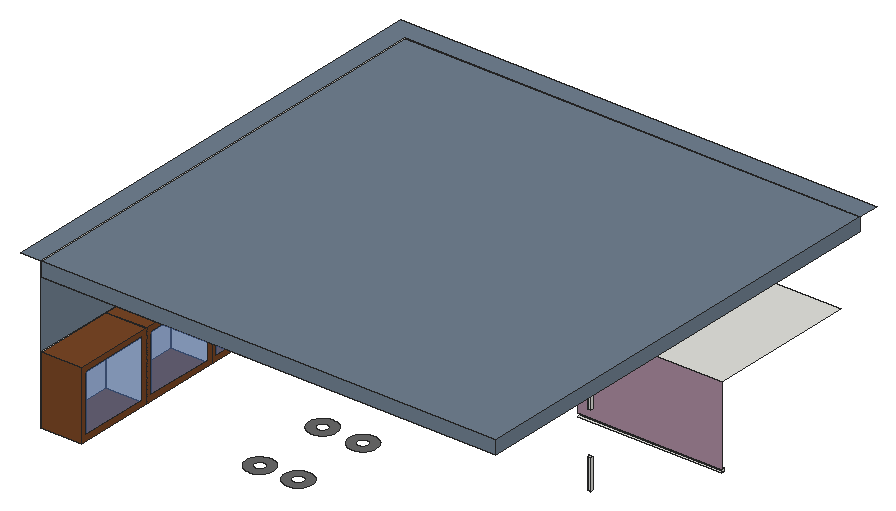
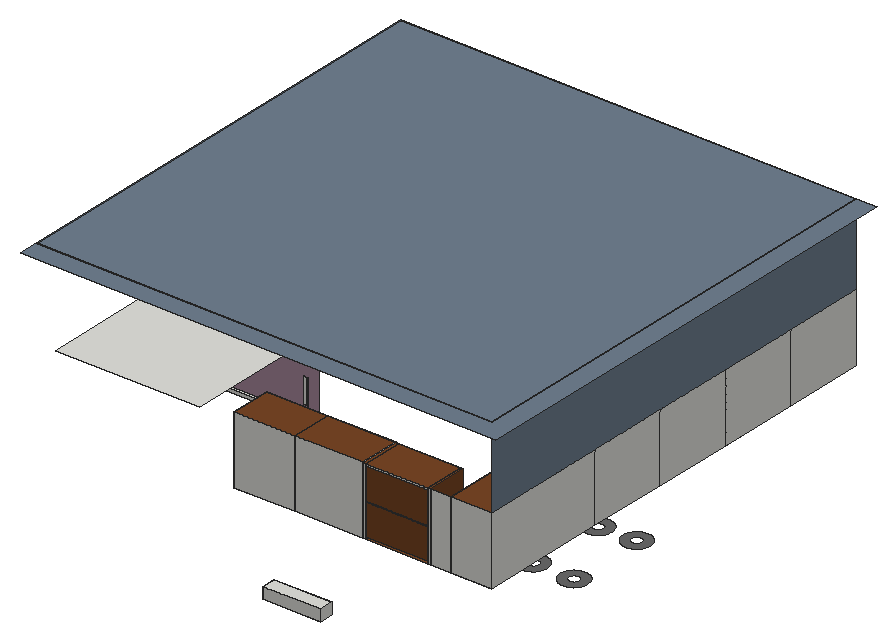
# SketchUp Ruby script. Lengths in inches.
U = 1.inch
M = Sketchup.active_model
def pt(a) = Geom::Point3d.new(a.map { |v| v * U })
def face(e, loops, mat)
  f = e.add_face(loops[0].map { |a| pt(a) })
  loops[1..].each { |l| e.add_face(l.map { |a| pt(a) }).erase! }
  f.material = f.back_material = mat if mat
  f
end
# faces: each face lists its corners as indices into pts; further lists are holes
def faces(e, pts, list, mat = nil) = list.each { |f| face(e, (f[0].is_a?(Array) ? f : [f]).map { |l| l.map { |i| pts[i] } }, mat) }
# xy, xz, yz: faces in a plane at the given z, y or x. An outline is a flat list of corners, or four numbers for a rectangle; further outlines are holes
def ring(l) = l.size == 4 ? [[l[0], l[1]], [l[2], l[1]], [l[2], l[3]], [l[0], l[3]]] : l.each_slice(2).to_a
def flat(e, list, mat, &to3) = list.each { |f| face(e, (f[0].is_a?(Array) ? f : [f]).map { |l| ring(l).map { |u, v| to3.(u, v) } }, mat) }
def xy(e, z, list, mat = nil) = flat(e, list, mat) { |x, y| [x, y, z] }
def xz(e, y, list, mat = nil) = flat(e, list, mat) { |x, z| [x, y, z] }
def yz(e, x, list, mat = nil) = flat(e, list, mat) { |y, z| [x, y, z] }
def lines(e, pts, list) = list.each { |a, b| e.add_line(pt(pts[a]), pt(pts[b])) }
# prism: a flat outline (further loops are holes) pulled along v
def prism(e, loops, v, mat = nil)
  f = face(e, loops, mat); d = Geom::Vector3d.new(v.map { |x| x * U })
  f.pushpull(f.normal.samedirection?(d) ? d.length : -d.length)
end
def box(e, o, s, mat = nil) = prism(e, [[o, [o[0] + s[0], o[1], o[2]], [o[0] + s[0], o[1] + s[1], o[2]], [o[0], o[1] + s[1], o[2]]]], [0, 0, s[2]], mat)
def at(x, y, z, deg = 0) = Geom::Transformation.translation(pt([x, y, z])) * Geom::Transformation.rotation(ORIGIN, Z_AXIS, deg.degrees)
def axes(o, x, y, z) = Geom::Transformation.new([*x, 0, *y, 0, *z, 0, *pt(o).to_a, 1])
def part(name) = M.definitions.add(name)
# library, detail: a bought-in or finely detailed component or shape, given as its bounding box
def library(name, o, s) = part(name).tap { |d| box(d.entities, o, s) }
def detail(e, o, s) = box(e.add_group.entities, o, s)
def put(e, d, t, mat = nil) = e.add_instance(d, t).tap { |i| i.material = mat if mat }
def group(e, t, mat = nil) = e.add_group.tap { |g| g.transformation = t; g.material = mat if mat }.entities
root = M.entities
M.materials.add("[0001_PaleVioletRed]").color = [219, 112, 147]
M.materials.add("[0004_HotPink]").color = [201, 82, 142]
M.materials.add("[0005_LightPink]").color = [255, 182, 193]
M.materials.add("[0111_SlateGray]").color = [112, 128, 144]
M.materials.add("[0134_DimGray]").color = [105, 105, 105]
M.materials.add("[Plywood]").color = [168, 138, 158]
M.materials.add("[Translucent Glass Blue]").color = [100, 149, 237]
M.materials["[Translucent Glass Blue]"].alpha = 0.5
M.materials.add("[Wood Veneer 01]").color = [120, 70, 37]
box(root,[169.29,389.375,124.83],[51.07,12.625,9.81])
xy(root,120,[[[75.05,157.99,76.31,158,77.56,158.13,78.78,158.4,79.98,158.8,81.12,159.32,82.2,159.95,83.21,160.7,84.14,161.55,84.98,162.48,85.71,163.51,86.33,164.6,86.83,165.75,87.21,166.95,87.46,168.18,87.59,169.43,87.58,170.68,87.44,171.93,87.17,173.16,86.77,174.35,86.26,175.49,85.62,176.58,84.875,177.59,84.03,178.52,83.09,179.35,82.07,180.08,80.98,180.7,79.83,181.21,78.63,181.59,77.4,181.84,76.15,181.96,74.89,181.95,73.64,181.8125,72.42,181.54,71.23,181.15,70.08,180.63,69,179.99,67.99,179.25,67.06,178.4,66.22,177.46,65.49,176.44,64.87,175.35,64.37,174.2,63.99,173,63.74,171.77,63.61,170.52,63.62,169.27,63.76,168.02,64.03,166.79,64.43,165.6,64.94,164.46,65.58,163.37,66.33,162.36,67.17,161.43,68.11,160.6,69.13,159.87,70.22,159.25,71.375,158.74,72.57,158.36,73.8,158.11],[75.77,164.98,75.25,164.99,74.73,165.05,74.22,165.17,73.73,165.34,73.25,165.56,72.8,165.83,72.39,166.14,72,166.5,71.66,166.9,71.36,167.32,71.11,167.78,70.9,168.26,70.75,168.76,70.65,169.28,70.6,169.8,70.61,170.32,70.68,170.84,70.79,171.35,70.96,171.85,71.19,172.32,71.45,172.77,71.77,173.1875,72.125,173.57,72.52,173.91,72.95,174.21,73.41,174.47,73.89,174.67,74.39,174.83,74.9,174.93,75.43,174.97,75.95,174.96,76.47,174.9,76.98,174.78,77.47,174.61,77.95,174.39,78.4,174.12,78.8125,173.8,79.2,173.45,79.54,173.05,79.84,172.625,80.09,172.17,80.3,171.68,80.45,171.18,80.55,170.67,80.6,170.15,80.59,169.625,80.52,169.11,80.41,168.6,80.24,168.1,80.01,167.625,79.75,167.18,79.43,166.76,79.07,166.38,78.68,166.03,78.25,165.73,77.79,165.48,77.31,165.28,76.81,165.12,76.3,165.02]],[[107.89,159.41,109.15,159.42,110.39,159.56,111.62,159.83,112.8125,160.22,113.96,160.74,115.04,161.375,116.05,162.12,116.98,162.97,117.8125,163.91,118.55,164.93,119.17,166.02,119.67,167.17,120.05,168.37,120.3,169.6,120.43,170.85,120.42,172.1,120.28,173.35,120.01,174.58,119.61,175.77,119.09,176.91,118.46,178,117.71,179.01,116.87,179.9375,115.93,180.77,114.91,181.5,113.81,182.125,112.66,182.625,111.47,183.01,110.24,183.26,108.99,183.38,107.73,183.375,106.48,183.23,105.26,182.97,104.0625,182.57,102.92,182.05,101.84,181.42,100.82,180.67,99.9,179.82,99.0625,178.88,98.33,177.86,97.71,176.77,97.21,175.62,96.83,174.42,96.57,173.19,96.45,171.94,96.46,170.6875,96.6,169.4375,96.87,168.21,97.26,167.02,97.78,165.875,98.42,164.79,99.16,163.78,100.01,162.85,100.95,162.02,101.97,161.29,103.0625,160.67,104.21,160.16,105.41,159.78,106.64,159.53],[108.61,166.4,108.09,166.41,107.57,166.47,107.06,166.59,106.57,166.76,106.09,166.98,105.64,167.25,105.22,167.57,104.84,167.92,104.5,168.32,104.2,168.75,103.94,169.2,103.74,169.69,103.59,170.1875,103.49,170.7,103.44,171.22,103.45,171.74,103.51,172.26,103.63,172.77,103.8,173.27,104.02,173.74,104.29,174.19,104.61,174.61,104.96,174.99,105.36,175.34,105.79,175.64,106.25,175.89,106.73,176.09,107.23,176.25,107.74,176.35,108.26,176.39,108.79,176.38,109.31,176.32,109.82,176.2,110.3125,176.03,110.79,175.81,111.23,175.54,111.65,175.23,112.03,174.87,112.38,174.47,112.68,174.04,112.93,173.59,113.14,173.11,113.29,172.6,113.39,172.09,113.44,171.57,113.43,171.05,113.36,170.53,113.24,170.02,113.07,169.52,112.85,169.05,112.58,168.6,112.27,168.18,111.91,167.8,111.52,167.46,111.09,167.16,110.63,166.9,110.15,166.7,109.65,166.54,109.13,166.44]],[[110.81,227.1,112.0625,227.11,113.31,227.25,114.54,227.52,115.73,227.91,116.875,228.43,117.96,229.07,118.97,229.8125,119.9,230.66,120.73,231.6,121.46,232.62,122.08,233.71,122.59,234.86,122.97,236.06,123.22,237.29,123.34,238.54,123.33,239.79,123.19,241.04,122.92,242.27,122.53,243.46,122.01,244.61,121.375,245.6875,120.63,246.7,119.78,247.63,118.84,248.46,117.82,249.19,116.73,249.81,115.58,250.32,114.38,250.7,113.15,250.95,111.9,251.07,110.65,251.07,109.4,250.93,108.17,250.66,106.98,250.26,105.83,249.74,104.75,249.11,103.74,248.36,102.8125,247.51,101.98,246.58,101.25,245.55,100.625,244.46,100.12,243.3125,99.74,242.11,99.49,240.88,99.37,239.63,99.375,238.38,99.51,237.13,99.78,235.9,100.18,234.71,100.7,233.57,101.33,232.48,102.08,231.47,102.93,230.54,103.86,229.71,104.89,228.98,105.98,228.36,107.13,227.85,108.33,227.47,109.56,227.22],[111.53,234.09,111.01,234.1,110.49,234.16,109.98,234.28,109.48,234.45,109.01,234.67,108.56,234.94,108.14,235.26,107.76,235.61,107.41,236.01,107.11,236.4375,106.86,236.89,106.66,237.375,106.5,237.875,106.4,238.39,106.36,238.91,106.37,239.44,106.43,239.95,106.55,240.46,106.72,240.96,106.9375,241.43,107.21,241.88,107.52,242.3,107.88,242.68,108.28,243.03,108.7,243.33,109.16,243.58,109.64,243.78,110.14,243.9375,110.66,244.04,111.18,244.08,111.7,244.07,112.22,244.01,112.73,243.89,113.23,243.72,113.7,243.5,114.15,243.23,114.57,242.92,114.95,242.56,115.29,242.16,115.59,241.74,115.85,241.28,116.05,240.8,116.21,240.3,116.31,239.78,116.35,239.26,116.34,238.74,116.28,238.22,116.16,237.71,115.99,237.21,115.77,236.74,115.5,236.29,115.18,235.87,114.83,235.49,114.43,235.15,114,234.85,113.55,234.59,113.0625,234.39,112.5625,234.23,112.05,234.14]],[[75.05,227.2,76.31,227.21,77.56,227.35,78.78,227.62,79.98,228.01,81.12,228.53,82.2,229.17,83.21,229.91,84.14,230.76,84.98,231.7,85.71,232.72,86.33,233.8125,86.83,234.96,87.21,236.16,87.46,237.39,87.59,238.64,87.58,239.9,87.44,241.14,87.17,242.37,86.77,243.5625,86.26,244.71,85.62,245.79,84.875,246.8,84.03,247.73,83.09,248.5625,82.07,249.3,80.98,249.92,79.83,250.42,78.63,250.8,77.4,251.05,76.15,251.18,74.89,251.17,73.64,251.03,72.42,250.76,71.23,250.36,70.08,249.84,69,249.21,67.99,248.46,67.06,247.62,66.22,246.68,65.49,245.66,64.87,244.5625,64.37,243.41,63.99,242.22,63.74,240.99,63.61,239.74,63.62,238.48,63.76,237.23,64.03,236,64.43,234.8125,64.94,233.67,65.58,232.58,66.33,231.57,67.17,230.65,68.11,229.8125,69.13,229.08,70.22,228.46,71.375,227.96,72.57,227.58,73.8,227.32],[75.77,234.19,75.25,234.2,74.73,234.26,74.22,234.38,73.73,234.55,73.25,234.77,72.8,235.04,72.39,235.36,72,235.71,71.66,236.11,71.36,236.54,71.11,237,70.9,237.48,70.75,237.98,70.65,238.49,70.6,239.01,70.61,239.54,70.68,240.06,70.79,240.57,70.96,241.0625,71.19,241.53,71.45,241.98,71.77,242.4,72.125,242.78,72.52,243.13,72.95,243.43,73.41,243.68,73.89,243.89,74.39,244.04,74.9,244.14,75.43,244.18,75.95,244.18,76.47,244.11,76.98,243.99,77.47,243.82,77.95,243.6,78.4,243.33,78.8125,243.02,79.2,242.66,79.54,242.27,79.84,241.84,80.09,241.38,80.3,240.9,80.45,240.4,80.55,239.88,80.6,239.36,80.59,238.84,80.52,238.32,80.41,237.81,80.24,237.31,80.01,236.84,79.75,236.39,79.43,235.97,79.07,235.59,78.68,235.25,78.25,234.95,77.79,234.69,77.31,234.49,76.81,234.34,76.3,234.24]]],"[0134_DimGray]")
xy(root,131.625,[[286.47,268,289.54,270]])
xy(root,158.25,[[286.47,268,289.54,270]])
xy(root,185.125,[[276,270,403.2,273]])
xy(root,188.125,[[276,270,403.2,273]])
xy(root,195.875,[[286.47,268,289.54,270]])
xy(root,204,[[18,0,54,72],[18,72,54,144],[18,144,54,216],[18,216,54,288],[18,288,54,402],
  [72,366,74.51,402],[74.51,366,129.17,402],[129.17,366,132,402],[132,366,192,402],[192,366,245.68,402]],"[Wood Veneer 01]")
xy(root,206,[[74.51,366,129.17,402]],"[Wood Veneer 01]")
xy(root,219.25,[[286.47,268,289.54,270]])
xy(root,233.33,[[74.51,366,129.17,402]],"[Wood Veneer 01]")
xy(root,234,[[74.51,366,129.17,402]],"[Wood Veneer 01]")
xy(root,257.125,[[276,270,403.2,402]])
xy(root,262,[[74.51,366,129.17,402]],"[Wood Veneer 01]")
xy(root,264,[[18,0,54,72],[18,72,54,144],[18,144,54,216],[18,216,54,288],[18,288,54,402],
  [72,366,74.51,402],[74.51,366,129.17,402],[129.17,366,132,402],[132,366,192,402],[192,366,245.68,402]],"[Wood Veneer 01]")
xy(root,324,[[386,60.51,385.37,60.52,384.75,60.6,384.14,60.74,383.54,60.95,382.97,61.22,382.4375,61.54,381.93,61.92,381.48,62.35,381.06,62.82,380.71,63.34,380.4,63.89,380.16,64.47,379.97,65.07,379.86,65.68,379.8,66.31,379.8125,66.9375,379.89,67.56,380.03,68.17,380.24,68.77,380.51,69.33,380.83,69.87,381.21,70.37,381.64,70.83,382.11,71.24,382.63,71.6,383.18,71.91,383.76,72.15,384.36,72.33,384.97,72.45,385.6,72.51,386.23,72.49,386.85,72.42,387.46,72.27,388.06,72.07,388.625,71.8,389.16,71.48,389.66,71.1,390.12,70.67,390.53,70.2,390.89,69.68,391.2,69.13,391.44,68.55,391.62,67.95,391.74,67.33,391.8,66.71,391.78,66.08,391.71,65.46,391.5625,64.85,391.36,64.25,391.09,63.68,390.77,63.15,390.39,62.64,389.96,62.1875,389.49,61.77,388.97,61.42,388.42,61.11,387.84,60.87,387.24,60.68,386.625,60.57],[60.5625,75.82,59.93,75.84,59.31,75.91,58.7,76.06,58.1,76.26,57.54,76.53,57,76.85,56.5,77.23,56.04,77.66,55.63,78.13,55.27,78.65,54.96,79.2,54.72,79.78,54.54,80.38,54.42,81,54.36,81.62,54.375,82.25,54.45,82.87,54.6,83.48,54.8,84.08,55.07,84.65,55.39,85.18,55.77,85.69,56.2,86.14,56.67,86.56,57.19,86.91,57.74,87.22,58.32,87.46,58.92,87.65,59.54,87.76,60.16,87.82,60.79,87.81,61.41,87.73,62.02,87.59,62.62,87.38,63.1875,87.11,63.72,86.79,64.23,86.41,64.68,85.98,65.1,85.51,65.45,84.99,65.76,84.44,66,83.86,66.19,83.26,66.3,82.65,66.36,82.02,66.35,81.39,66.27,80.77,66.125,80.16,65.92,79.56,65.65,79,65.33,78.46,64.95,77.96,64.52,77.5,64.05,77.09,63.53,76.73,62.98,76.42,62.4,76.18,61.8,76,61.1875,75.88],[57.37,156.57,56.74,156.59,56.12,156.66,55.51,156.81,54.91,157.01,54.34,157.28,53.81,157.6,53.31,157.98,52.85,158.41,52.44,158.88,52.08,159.4,51.77,159.95,51.53,160.53,51.35,161.13,51.23,161.75,51.17,162.37,51.18,163,51.26,163.62,51.4,164.23,51.61,164.83,51.875,165.4,52.2,165.93,52.58,166.44,53.01,166.89,53.48,167.31,54,167.66,54.55,167.97,55.125,168.21,55.73,168.4,56.34,168.51,56.97,168.57,57.6,168.56,58.22,168.48,58.83,168.34,59.43,168.13,59.99,167.86,60.53,167.54,61.03,167.16,61.49,166.73,61.9,166.26,62.26,165.74,62.57,165.19,62.8125,164.61,62.99,164.01,63.11,163.4,63.17,162.77,63.15,162.14,63.08,161.52,62.93,160.91,62.73,160.31,62.46,159.75,62.14,159.21,61.76,158.71,61.33,158.25,60.86,157.84,60.34,157.48,59.79,157.17,59.21,156.93,58.61,156.75,57.99,156.63],[386,156.57,385.37,156.59,384.75,156.66,384.14,156.81,383.54,157.01,382.97,157.28,382.4375,157.6,381.93,157.98,381.48,158.41,381.06,158.88,380.71,159.4,380.4,159.95,380.16,160.53,379.97,161.13,379.86,161.75,379.8,162.37,379.8125,163,379.89,163.62,380.03,164.23,380.24,164.83,380.51,165.4,380.83,165.93,381.21,166.44,381.64,166.89,382.11,167.31,382.63,167.66,383.18,167.97,383.76,168.21,384.36,168.4,384.97,168.51,385.6,168.57,386.23,168.56,386.85,168.48,387.46,168.34,388.06,168.13,388.625,167.86,389.16,167.54,389.66,167.16,390.12,166.73,390.53,166.26,390.89,165.74,391.2,165.19,391.44,164.61,391.62,164.01,391.74,163.4,391.8,162.77,391.78,162.14,391.71,161.52,391.5625,160.91,391.36,160.31,391.09,159.75,390.77,159.21,390.39,158.71,389.96,158.25,389.49,157.84,388.97,157.48,388.42,157.17,387.84,156.93,387.24,156.75,386.625,156.63],[60.5625,254.01,59.93,254.02,59.31,254.1,58.7,254.24,58.1,254.45,57.54,254.72,57,255.04,56.5,255.42,56.04,255.85,55.63,256.32,55.27,256.84,54.96,257.39,54.72,257.97,54.54,258.57,54.42,259.18,54.36,259.81,54.375,260.4375,54.45,261.06,54.6,261.67,54.8,262.27,55.07,262.83,55.39,263.37,55.77,263.87,56.2,264.33,56.67,264.74,57.19,265.1,57.74,265.41,58.32,265.65,58.92,265.83,59.54,265.95,60.16,266.01,60.79,265.99,61.41,265.92,62.02,265.77,62.62,265.57,63.1875,265.3,63.72,264.98,64.23,264.6,64.68,264.17,65.1,263.7,65.45,263.18,65.76,262.63,66,262.05,66.19,261.45,66.3,260.83,66.36,260.21,66.35,259.58,66.27,258.96,66.125,258.35,65.92,257.75,65.65,257.18,65.33,256.65,64.95,256.14,64.52,255.6875,64.05,255.27,63.53,254.92,62.98,254.61,62.4,254.37,61.8,254.18,61.1875,254.07],
  [386,254.01,385.37,254.02,384.75,254.1,384.14,254.24,383.54,254.45,382.97,254.72,382.4375,255.04,381.93,255.42,381.48,255.85,381.06,256.32,380.71,256.84,380.4,257.39,380.16,257.97,379.97,258.57,379.86,259.18,379.8,259.81,379.8125,260.4375,379.89,261.06,380.03,261.67,380.24,262.27,380.51,262.83,380.83,263.37,381.21,263.87,381.64,264.33,382.11,264.74,382.63,265.1,383.18,265.41,383.76,265.65,384.36,265.83,384.97,265.95,385.6,266.01,386.23,265.99,386.85,265.92,387.46,265.77,388.06,265.57,388.625,265.3,389.16,264.98,389.66,264.6,390.12,264.17,390.53,263.7,390.89,263.18,391.2,262.63,391.44,262.05,391.62,261.45,391.74,260.83,391.8,260.21,391.78,259.58,391.71,258.96,391.5625,258.35,391.36,257.75,391.09,257.18,390.77,256.65,390.39,256.14,389.96,255.6875,389.49,255.27,388.97,254.92,388.42,254.61,387.84,254.37,387.24,254.18,386.625,254.07]])
xy(root,324,[[116.88,86.3,115.35,86.4,113.85,86.7,112.4,87.1875,111.02,87.87,109.75,88.72,108.6,89.73,107.59,90.88,106.74,92.15,106.06,93.53,105.56,94.98,105.27,96.48,105.17,98.01,105.17,298.06,105.36,301.03,105.94,303.95,106.9,306.77,108.21,309.4375,109.87,311.92,111.83,314.15,114.07,316.12,116.55,317.77,119.22,319.09,122.04,320.04,124.96,320.625,127.93,320.82,322.53,320.82,324.77,320.67,326.97,320.24,329.09,319.51,331.11,318.52,332.97,317.27,334.66,315.79,336.14,314.11,337.39,312.24,338.38,310.23,339.1,308.1,339.54,305.9,339.6875,303.66,339.6875,98.17,339.59,96.62,339.28,95.1,338.78,93.63,338.1,92.23,337.23,90.94,336.21,89.78,335.04,88.75,333.75,87.89,332.36,87.2,330.89,86.7,329.36,86.4,327.8125,86.3]],"[0004_HotPink]")
xy(root,324,[[[18,0,420,402],[116.88,75.03,327.8125,75.03,330.83,75.23,333.8,75.82,336.67,76.79,339.39,78.13,341.9,79.81,344.18,81.81,346.18,84.08,347.86,86.6,349.2,89.31,350.17,92.18,350.76,95.15,350.96,98.17,350.96,303.66,350.71,307.37,349.99,311.02,348.79,314.54,347.15,317.875,345.08,320.97,342.63,323.76,339.83,326.21,336.74,328.28,333.41,329.93,329.88,331.12,326.24,331.85,322.53,332.09,127.93,332.09,123.48,331.8,119.12,330.93,114.9,329.5,110.91,327.53,107.21,325.06,103.86,322.12,100.93,318.78,98.46,315.07,96.49,311.08,95.06,306.87,94.1875,302.5,93.9,298.06,93.9,98.01,94.09,95.01,94.68,92.0625,95.65,89.22,96.98,86.52,98.65,84.02,100.63,81.76,102.89,79.78,105.39,78.11,108.08,76.78,110.93,75.8125,113.88,75.22],[386,156.57,386.625,156.63,387.24,156.75,387.84,156.93,388.42,157.17,388.97,157.48,389.49,157.84,389.96,158.25,390.39,158.71,390.77,159.21,391.09,159.75,391.36,160.31,391.5625,160.91,391.71,161.52,391.78,162.14,391.8,162.77,391.74,163.4,391.62,164.01,391.44,164.61,391.2,165.19,390.89,165.74,390.53,166.26,390.12,166.73,389.66,167.16,389.16,167.54,388.625,167.86,388.06,168.13,387.46,168.34,386.85,168.48,386.23,168.56,385.6,168.57,384.97,168.51,384.36,168.4,383.76,168.21,383.18,167.97,382.63,167.66,382.11,167.31,381.64,166.89,381.21,166.44,380.83,165.93,380.51,165.4,380.24,164.83,380.03,164.23,379.89,163.62,379.8125,163,379.8,162.37,379.86,161.75,379.97,161.13,380.16,160.53,380.4,159.95,380.71,159.4,381.06,158.88,381.48,158.41,381.93,157.98,382.4375,157.6,382.97,157.28,383.54,157.01,384.14,156.81,384.75,156.66,385.37,156.59],[57.37,156.57,57.99,156.63,58.61,156.75,59.21,156.93,59.79,157.17,60.34,157.48,60.86,157.84,61.33,158.25,61.76,158.71,62.14,159.21,62.46,159.75,62.73,160.31,62.93,160.91,63.08,161.52,63.15,162.14,63.17,162.77,63.11,163.4,62.99,164.01,62.8125,164.61,62.57,165.19,62.26,165.74,61.9,166.26,61.49,166.73,61.03,167.16,60.53,167.54,59.99,167.86,59.43,168.13,58.83,168.34,58.22,168.48,57.6,168.56,56.97,168.57,56.34,168.51,55.73,168.4,55.125,168.21,54.55,167.97,54,167.66,53.48,167.31,53.01,166.89,52.58,166.44,52.2,165.93,51.875,165.4,51.61,164.83,51.4,164.23,51.26,163.62,51.18,163,51.17,162.37,51.23,161.75,51.35,161.13,51.53,160.53,51.77,159.95,52.08,159.4,52.44,158.88,52.85,158.41,53.31,157.98,53.81,157.6,54.34,157.28,54.91,157.01,55.51,156.81,56.12,156.66,56.74,156.59],[386,60.51,386.625,60.57,387.24,60.68,387.84,60.87,388.42,61.11,388.97,61.42,389.49,61.77,389.96,62.1875,390.39,62.64,390.77,63.15,391.09,63.68,391.36,64.25,391.5625,64.85,391.71,65.46,391.78,66.08,391.8,66.71,391.74,67.33,391.62,67.95,391.44,68.55,391.2,69.13,390.89,69.68,390.53,70.2,390.12,70.67,389.66,71.1,389.16,71.48,388.625,71.8,388.06,72.07,387.46,72.27,386.85,72.42,386.23,72.49,385.6,72.51,384.97,72.45,384.36,72.33,383.76,72.15,383.18,71.91,382.63,71.6,382.11,71.24,381.64,70.83,381.21,70.37,380.83,69.87,380.51,69.33,380.24,68.77,380.03,68.17,379.89,67.56,379.8125,66.9375,379.8,66.31,379.86,65.68,379.97,65.07,380.16,64.47,380.4,63.89,380.71,63.34,381.06,62.82,381.48,62.35,381.93,61.92,382.4375,61.54,382.97,61.22,383.54,60.95,384.14,60.74,384.75,60.6,385.37,60.52],[386,254.01,386.625,254.07,387.24,254.18,387.84,254.37,388.42,254.61,388.97,254.92,389.49,255.27,389.96,255.6875,390.39,256.14,390.77,256.65,391.09,257.18,391.36,257.75,391.5625,258.35,391.71,258.96,391.78,259.58,391.8,260.21,391.74,260.83,391.62,261.45,391.44,262.05,391.2,262.63,390.89,263.18,390.53,263.7,390.12,264.17,389.66,264.6,389.16,264.98,388.625,265.3,388.06,265.57,387.46,265.77,386.85,265.92,386.23,265.99,385.6,266.01,384.97,265.95,384.36,265.83,383.76,265.65,383.18,265.41,382.63,265.1,382.11,264.74,381.64,264.33,381.21,263.87,380.83,263.37,380.51,262.83,380.24,262.27,380.03,261.67,379.89,261.06,379.8125,260.4375,379.8,259.81,379.86,259.18,379.97,258.57,380.16,257.97,380.4,257.39,380.71,256.84,381.06,256.32,381.48,255.85,381.93,255.42,382.4375,255.04,382.97,254.72,383.54,254.45,384.14,254.24,384.75,254.1,385.37,254.02],[60.5625,254.01,61.1875,254.07,61.8,254.18,62.4,254.37,62.98,254.61,63.53,254.92,64.05,255.27,64.52,255.6875,64.95,256.14,65.33,256.65,65.65,257.18,65.92,257.75,66.125,258.35,66.27,258.96,66.35,259.58,66.36,260.21,66.3,260.83,66.19,261.45,66,262.05,65.76,262.63,65.45,263.18,65.1,263.7,64.68,264.17,64.23,264.6,63.72,264.98,63.1875,265.3,62.62,265.57,62.02,265.77,61.41,265.92,60.79,265.99,60.16,266.01,59.54,265.95,58.92,265.83,58.32,265.65,57.74,265.41,57.19,265.1,56.67,264.74,56.2,264.33,55.77,263.87,55.39,263.37,55.07,262.83,54.8,262.27,54.6,261.67,54.45,261.06,54.375,260.4375,54.36,259.81,54.42,259.18,54.54,258.57,54.72,257.97,54.96,257.39,55.27,256.84,55.63,256.32,56.04,255.85,56.5,255.42,57,255.04,57.54,254.72,58.1,254.45,58.7,254.24,59.31,254.1,59.93,254.02],[60.5625,75.82,61.1875,75.88,61.8,76,62.4,76.18,62.98,76.42,63.53,76.73,64.05,77.09,64.52,77.5,64.95,77.96,65.33,78.46,65.65,79,65.92,79.56,66.125,80.16,66.27,80.77,66.35,81.39,66.36,82.02,66.3,82.65,66.19,83.26,66,83.86,65.76,84.44,65.45,84.99,65.1,85.51,64.68,85.98,64.23,86.41,63.72,86.79,63.1875,87.11,62.62,87.38,62.02,87.59,61.41,87.73,60.79,87.81,60.16,87.82,59.54,87.76,58.92,87.65,58.32,87.46,57.74,87.22,57.19,86.91,56.67,86.56,56.2,86.14,55.77,85.69,55.39,85.18,55.07,84.65,54.8,84.08,54.6,83.48,54.45,82.87,54.375,82.25,54.36,81.62,54.42,81,54.54,80.38,54.72,79.78,54.96,79.2,55.27,78.65,55.63,78.13,56.04,77.66,56.5,77.23,57,76.85,57.54,76.53,58.1,76.26,58.7,76.06,59.31,75.91,59.93,75.84]]],"[0005_LightPink]")
xy(root,328,[[[116.88,75.03,113.88,75.22,110.93,75.8125,108.08,76.78,105.39,78.11,102.89,79.78,100.63,81.76,98.65,84.02,96.98,86.52,95.65,89.22,94.68,92.0625,94.09,95.01,93.9,98.01,93.9,298.06,94.1875,302.5,95.06,306.87,96.49,311.08,98.46,315.07,100.93,318.78,103.86,322.12,107.21,325.06,110.91,327.53,114.9,329.5,119.12,330.93,123.48,331.8,127.93,332.09,322.53,332.09,326.24,331.85,329.88,331.12,333.41,329.93,336.74,328.28,339.83,326.21,342.63,323.76,345.08,320.97,347.15,317.875,348.79,314.54,349.99,311.02,350.71,307.37,350.96,303.66,350.96,98.17,350.76,95.15,350.17,92.18,349.2,89.31,347.86,86.6,346.18,84.08,344.18,81.81,341.9,79.81,339.39,78.13,336.67,76.79,333.8,75.82,330.83,75.23,327.8125,75.03],[116.88,86.3,327.8125,86.3,329.36,86.4,330.89,86.7,332.36,87.2,333.75,87.89,335.04,88.75,336.21,89.78,337.23,90.94,338.1,92.23,338.78,93.63,339.28,95.1,339.59,96.62,339.6875,98.17,339.6875,303.66,339.54,305.9,339.1,308.1,338.38,310.23,337.39,312.24,336.14,314.11,334.66,315.79,332.97,317.27,331.11,318.52,329.09,319.51,326.97,320.24,324.77,320.67,322.53,320.82,127.93,320.82,124.96,320.625,122.04,320.04,119.22,319.09,116.55,317.77,114.07,316.12,111.83,314.15,109.87,311.92,108.21,309.4375,106.9,306.77,105.94,303.95,105.36,301.03,105.17,298.06,105.17,98.01,105.27,96.48,105.56,94.98,106.06,93.53,106.74,92.15,107.59,90.88,108.6,89.73,109.75,88.72,111.02,87.87,112.4,87.1875,113.85,86.7,115.35,86.4]]],"[0001_PaleVioletRed]")
xy(root,336,[[0,0,18,0,18,402,420,402,420,420,0,420],[18,0,420,402]],"[0111_SlateGray]")
xz(root,0,[[18,324,420,336]],"[0111_SlateGray]")
xz(root,0,[[18,204,54,264]],"[Wood Veneer 01]")
xz(root,72,[[18,204,54,264]])
xz(root,75.03,[[116.88,324,327.8125,328]],"[0001_PaleVioletRed]")
xz(root,86.3,[[116.88,324,327.8125,328]],"[0004_HotPink]")
xz(root,144,[[18,204,54,264]])
xz(root,216,[[18,204,54,264]])
xz(root,268,[[286.47,131.625,289.54,158.25],[286.47,195.875,289.54,219.25]])
xz(root,270,[[[276,188.125,403.2,257.125],[286.47,195.875,289.54,219.25]]],"[Plywood]")
xz(root,273,[[276,185.125,403.2,188.125]])
xz(root,288,[[18,204,54,264]])
xz(root,320.82,[[127.93,324,322.53,328]],"[0004_HotPink]")
xz(root,332.09,[[127.93,324,322.53,328]],"[0001_PaleVioletRed]")
xz(root,366,[[74.51,206,129.17,233.33],[135.21,207.21,188.79,260.79],[195.21,207.21,242.47,260.79],[74.51,234,129.17,262]],"[Translucent Glass Blue]")
xz(root,366,[[72,204,74.51,264],[74.51,204,129.17,206],[129.17,204,132,264],[[132,204,192,264],[135.21,207.21,188.79,260.79]],[[192,204,245.68,264],[195.21,207.21,242.47,260.79]],
  [74.51,233.33,129.17,234],[74.51,262,129.17,264]],"[Wood Veneer 01]")
xz(root,402,[[18,204,54,264],[54,204,72,264],[72,204,74.51,264],[129.17,204,132,264],[132,204,192,264],
  [192,204,245.68,264],[74.51,233.33,129.17,234],[74.51,262,129.17,264],[18,324,420,336]])
xz(root,402,[[74.51,206,129.17,233.33],[74.51,234,129.17,262]],"[Wood Veneer 01]")
yz(root,18,[[0,204,72,264],[72,204,144,264],[144,204,216,264],[216,204,288,264],[288,204,402,264],
  [0,324,402,336]])
yz(root,18,[[0,264,402,324]],"[0111_SlateGray]")
yz(root,54,[[4.86,208.86,67.14,259.14],[76.86,208.86,139.14,259.14],[148.86,208.86,211.14,259.14],[220.86,208.86,283.14,259.14],[292.86,208.86,397.14,259.14]],"[Translucent Glass Blue]")
yz(root,54,[[[0,204,72,264],[4.86,208.86,67.14,259.14]],[[72,204,144,264],[76.86,208.86,139.14,259.14]],[[144,204,216,264],[148.86,208.86,211.14,259.14]],[[216,204,288,264],[220.86,208.86,283.14,259.14]],[[288,204,402,264],[292.86,208.86,397.14,259.14]]],"[Wood Veneer 01]")
yz(root,72,[[366,204,402,264]],"[Wood Veneer 01]")
yz(root,74.51,[[366,204,402,206],[366,233.33,402,234],[366,262,402,264]])
yz(root,74.51,[[366,206,402,233.33],[366,234,402,262]],"[Wood Veneer 01]")
yz(root,93.9,[[98.01,324,298.06,328]],"[0001_PaleVioletRed]")
yz(root,105.17,[[98.01,324,298.06,328]],"[0004_HotPink]")
yz(root,129.17,[[366,204,402,206],[366,233.33,402,234],[366,262,402,264]])
yz(root,129.17,[[366,206,402,233.33],[366,234,402,262]],"[Wood Veneer 01]")
yz(root,132,[[366,204,402,264]])
yz(root,192,[[366,204,402,264]])
yz(root,245.68,[[366,204,402,264]],"[Wood Veneer 01]")
yz(root,286.47,[[268,131.625,270,158.25],[268,195.875,270,219.25]])
yz(root,289.54,[[268,131.625,270,158.25],[268,195.875,270,219.25]])
yz(root,339.6875,[[98.17,324,303.66,328]],"[0004_HotPink]")
yz(root,350.96,[[98.17,324,303.66,328]],"[0001_PaleVioletRed]")
yz(root,420,[[0,324,402,336]],"[0111_SlateGray]")
p = [[116.88,75.03,324],[113.88,75.22,324],[113.88,75.22,328],[116.88,75.03,328],[330.83,75.23,324],[327.8125,75.03,324],
  [327.8125,75.03,328],[330.83,75.23,328],[110.93,75.8125,324],[110.93,75.8125,328],[333.8,75.82,324],[333.8,75.82,328],
  [108.08,76.78,324],[108.08,76.78,328],[336.67,76.79,324],[336.67,76.79,328],[105.39,78.11,324],[105.39,78.11,328],
  [339.39,78.13,324],[339.39,78.13,328],[102.89,79.78,324],[102.89,79.78,328],[341.9,79.81,324],[341.9,79.81,328],
  [100.63,81.76,324],[100.63,81.76,328],[344.18,81.81,324],[344.18,81.81,328],[98.65,84.02,324],[98.65,84.02,328],
  [346.18,84.08,324],[346.18,84.08,328],[96.98,86.52,324],[96.98,86.52,328],[347.86,86.6,324],[347.86,86.6,328],
  [115.35,86.4,324],[116.88,86.3,324],[116.88,86.3,328],[115.35,86.4,328],[327.8125,86.3,324],[329.36,86.4,324],
  [329.36,86.4,328],[327.8125,86.3,328],[113.85,86.7,324],[113.85,86.7,328],[330.89,86.7,324],[330.89,86.7,328],
  [95.65,89.22,324],[95.65,89.22,328],[349.2,89.31,324],[349.2,89.31,328],[112.4,87.1875,324],[112.4,87.1875,328],
  [332.36,87.2,324],[332.36,87.2,328],[111.02,87.87,324],[111.02,87.87,328],[333.75,87.89,324],[333.75,87.89,328],
  [109.75,88.72,324],[109.75,88.72,328],[335.04,88.75,324],[335.04,88.75,328],[108.6,89.73,324],[108.6,89.73,328],
  [336.21,89.78,324],[336.21,89.78,328],[94.68,92.0625,324],[94.68,92.0625,328],[350.17,92.18,324],[350.17,92.18,328],
  [107.59,90.88,324],[107.59,90.88,328],[337.23,90.94,324],[337.23,90.94,328],[106.74,92.15,324],[106.74,92.15,328],
  [338.1,92.23,324],[338.1,92.23,328],[94.09,95.01,324],[94.09,95.01,328],[106.06,93.53,324],[106.06,93.53,328],
  [338.78,93.63,324],[338.78,93.63,328],[350.76,95.15,324],[350.76,95.15,328],[105.56,94.98,324],[105.56,94.98,328],
  [339.28,95.1,324],[339.28,95.1,328],[93.9,98.01,324],[93.9,98.01,328],[105.27,96.48,324],[105.27,96.48,328],
  [339.59,96.62,324],[339.59,96.62,328],[350.96,98.17,324],[350.96,98.17,328],[105.17,98.01,324],[105.17,98.01,328],
  [339.6875,98.17,324],[339.6875,98.17,328],[93.9,298.06,324],[94.1875,302.5,324],[94.1875,302.5,328],[93.9,298.06,328],
  [105.36,301.03,324],[105.17,298.06,324],[105.17,298.06,328],[105.36,301.03,328],[105.94,303.95,324],[105.94,303.95,328],
  [95.06,306.87,324],[95.06,306.87,328],[339.6875,303.66,324],[339.54,305.9,324],[339.54,305.9,328],[339.6875,303.66,328],
  [350.71,307.37,324],[350.96,303.66,324],[350.96,303.66,328],[350.71,307.37,328],[106.9,306.77,324],[106.9,306.77,328],
  [339.1,308.1,324],[339.1,308.1,328],[108.21,309.4375,324],[108.21,309.4375,328],[96.49,311.08,324],[96.49,311.08,328],
  [349.99,311.02,324],[349.99,311.02,328],[338.38,310.23,324],[338.38,310.23,328],[109.87,311.92,324],[109.87,311.92,328],
  [337.39,312.24,324],[337.39,312.24,328],[348.79,314.54,324],[348.79,314.54,328],[98.46,315.07,324],[98.46,315.07,328],
  [111.83,314.15,324],[111.83,314.15,328],[336.14,314.11,324],[336.14,314.11,328],[334.66,315.79,324],[334.66,315.79,328],
  [114.07,316.12,324],[114.07,316.12,328],[347.15,317.875,324],[347.15,317.875,328],[100.93,318.78,324],[100.93,318.78,328],
  [332.97,317.27,324],[332.97,317.27,328],[116.55,317.77,324],[116.55,317.77,328],[331.11,318.52,324],[331.11,318.52,328],
  [119.22,319.09,324],[119.22,319.09,328],[345.08,320.97,324],[345.08,320.97,328],[329.09,319.51,324],[329.09,319.51,328],
  [103.86,322.12,324],[103.86,322.12,328],[122.04,320.04,324],[122.04,320.04,328],[326.97,320.24,324],[326.97,320.24,328],
  [124.96,320.625,324],[124.96,320.625,328],[324.77,320.67,324],[324.77,320.67,328],[127.93,320.82,324],[127.93,320.82,328],
  [322.53,320.82,324],[322.53,320.82,328],[342.63,323.76,324],[342.63,323.76,328],[107.21,325.06,324],[107.21,325.06,328],
  [339.83,326.21,324],[339.83,326.21,328],[110.91,327.53,324],[110.91,327.53,328],[336.74,328.28,324],[336.74,328.28,328],
  [114.9,329.5,324],[114.9,329.5,328],[333.41,329.93,324],[333.41,329.93,328],[119.12,330.93,324],[119.12,330.93,328],
  [329.88,331.12,324],[329.88,331.12,328],[123.48,331.8,324],[123.48,331.8,328],[326.24,331.85,324],[326.24,331.85,328],
  [127.93,332.09,324],[127.93,332.09,328],[322.53,332.09,324],[322.53,332.09,328]]
faces(root,p,[[0,1,2,3],[4,5,6,7],[1,8,9,2],[10,4,7,11],[8,12,13,9],[14,10,11,15],[12,16,17,13],[18,14,15,19],
  [16,20,21,17],[22,18,19,23],[20,24,25,21],[26,22,23,27],[24,28,29,25],[30,26,27,31],[28,32,33,29],[34,30,31,35],
  [32,48,49,33],[50,34,35,51],[48,68,69,49],[70,50,51,71],[68,80,81,69],[86,70,71,87],[80,92,93,81],[98,86,87,99],
  [104,105,106,107],[105,114,115,106],[120,121,122,123],[114,130,131,115],[132,120,123,133],[140,132,133,141],[130,142,143,131],[152,140,141,153],
  [142,154,155,143],[164,152,153,165],[154,168,169,155],[182,164,165,183],[168,184,185,169],[186,182,183,187],[184,188,189,185],[190,186,187,191],
  [188,192,193,189],[194,190,191,195],[192,196,197,193],[198,194,195,199],[196,200,201,197],[202,198,199,203],[200,204,205,201],[206,202,203,207]],"[0001_PaleVioletRed]")
faces(root,p,[[36,37,38,39],[40,41,42,43],[44,36,39,45],[41,46,47,42],[52,44,45,53],[46,54,55,47],[56,52,53,57],[54,58,59,55],
  [60,56,57,61],[58,62,63,59],[64,60,61,65],[62,66,67,63],[72,64,65,73],[66,74,75,67],[76,72,73,77],[74,78,79,75],
  [82,76,77,83],[78,84,85,79],[88,82,83,89],[84,90,91,85],[94,88,89,95],[90,96,97,91],[100,94,95,101],[96,102,103,97],
  [116,117,118,119],[117,126,127,118],[126,134,135,127],[134,138,139,135],[138,146,147,139],[146,148,149,147],[148,156,157,149],[156,160,161,157],
  [160,166,167,161],[166,172,173,167],[172,176,177,173],[176,180,181,177]],"[0004_HotPink]")
faces(root,p,[[108,109,110,111],[112,108,111,113],[124,112,113,125],[128,124,125,129],[136,128,129,137],[144,136,137,145],[150,144,145,151],[158,150,151,159],
  [162,158,159,163],[170,162,163,171],[174,170,171,175],[178,174,175,179]])
